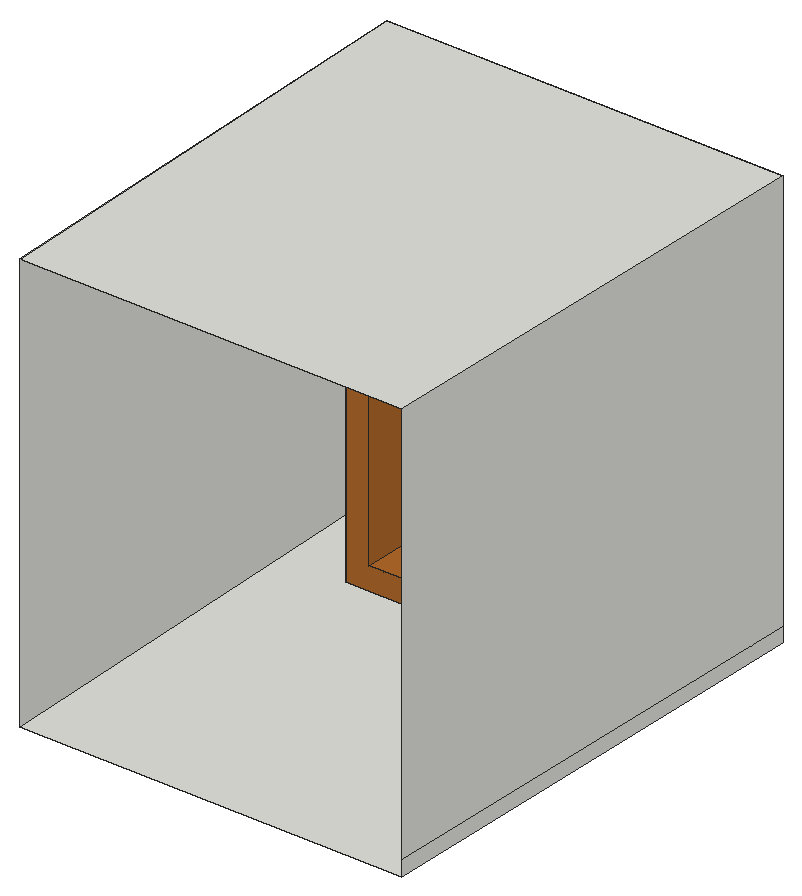
# SketchUp Ruby script. Lengths in inches.
U = 1.inch
M = Sketchup.active_model
def pt(a) = Geom::Point3d.new(a.map { |v| v * U })
def face(e, loops, mat)
  f = e.add_face(loops[0].map { |a| pt(a) })
  loops[1..].each { |l| e.add_face(l.map { |a| pt(a) }).erase! }
  f.material = f.back_material = mat if mat
  f
end
# faces: each face lists its corners as indices into pts; further lists are holes
def faces(e, pts, list, mat = nil) = list.each { |f| face(e, (f[0].is_a?(Array) ? f : [f]).map { |l| l.map { |i| pts[i] } }, mat) }
# xy, xz, yz: faces in a plane at the given z, y or x. An outline is a flat list of corners, or four numbers for a rectangle; further outlines are holes
def ring(l) = l.size == 4 ? [[l[0], l[1]], [l[2], l[1]], [l[2], l[3]], [l[0], l[3]]] : l.each_slice(2).to_a
def flat(e, list, mat, &to3) = list.each { |f| face(e, (f[0].is_a?(Array) ? f : [f]).map { |l| ring(l).map { |u, v| to3.(u, v) } }, mat) }
def xy(e, z, list, mat = nil) = flat(e, list, mat) { |x, y| [x, y, z] }
def xz(e, y, list, mat = nil) = flat(e, list, mat) { |x, z| [x, y, z] }
def yz(e, x, list, mat = nil) = flat(e, list, mat) { |y, z| [x, y, z] }
def lines(e, pts, list) = list.each { |a, b| e.add_line(pt(pts[a]), pt(pts[b])) }
# prism: a flat outline (further loops are holes) pulled along v
def prism(e, loops, v, mat = nil)
  f = face(e, loops, mat); d = Geom::Vector3d.new(v.map { |x| x * U })
  f.pushpull(f.normal.samedirection?(d) ? d.length : -d.length)
end
def box(e, o, s, mat = nil) = prism(e, [[o, [o[0] + s[0], o[1], o[2]], [o[0] + s[0], o[1] + s[1], o[2]], [o[0], o[1] + s[1], o[2]]]], [0, 0, s[2]], mat)
def at(x, y, z, deg = 0) = Geom::Transformation.translation(pt([x, y, z])) * Geom::Transformation.rotation(ORIGIN, Z_AXIS, deg.degrees)
def axes(o, x, y, z) = Geom::Transformation.new([*x, 0, *y, 0, *z, 0, *pt(o).to_a, 1])
def part(name) = M.definitions.add(name)
# library, detail: a bought-in or finely detailed component or shape, given as its bounding box
def library(name, o, s) = part(name).tap { |d| box(d.entities, o, s) }
def detail(e, o, s) = box(e.add_group.entities, o, s)
def put(e, d, t, mat = nil) = e.add_instance(d, t).tap { |i| i.material = mat if mat }
def group(e, t, mat = nil) = e.add_group.tap { |g| g.transformation = t; g.material = mat if mat }.entities
root = M.entities
M.materials.add("[Field Square Tile]").color = [217, 201, 169]
M.materials.add("[Mirror 02]").color = [229, 229, 229]
M.materials.add("[Wood Bamboo]").color = [177, 105, 43]
M.materials.add("[Wood Floor Parquet]").color = [145, 89, 39]
c1 = part("Group19\#1")
p = [[0,0,0],[0,0,-10.8125],[-3.6875,0,-10.8125],[24,-11,0],[-24,-11,0],[24,11,0],
  [24,0,0],[-24,11,0],[3.6875,0,-10.8125],[-24,0,0],[0,0,-17.5]]
lines(c1.entities,p,[[0,1],[1,2],[3,4],[5,6],[7,5],[1,8],[9,0],[0,6],[8,10],[4,9],[6,3],[2,10],
  [9,7]])
c2 = part("Rectangle Light")
put(c2.entities,c1,at(0,0,0))
c3 = part("Timber post")
box(c3.entities,[0,-2,0],[2,2,84],"[Wood Bamboo]")
c4 = part("Group\#13")
put(c4.entities,c3,at(0,0,0))
c5 = library("Group\#4",[0,0,0],[15,0.9,42])
c6 = library("Group\#5",[0,0,0],[15,0.9,60])
xy(root,-6,[[3.67,0,104.23,0,104.23,125.21,0,125.21]])
xy(root,104.23,[[3.67,0,0,125.21,104.23,125.21,104.23,0]])
xz(root,125.21,[[0,-6,104.23,104.23]])
yz(root,104.23,[[0,-6,125.21,-2.16],[0,-2.16,125.21,104.23]])
p = [[3.67,0,-6],[0,125.21,-6],[0,125.21,104.23],[3.67,0,104.23]]
faces(root,p,[[0,1,2,3]])
g1 = group(root,at(24.24,113.14,0))
box(g1,[0,2,0],[48,2,84])
xz(g1,0,[[0,0,2,84],[2,0,47.75,84],[47.75,0,48,84]])
g2 = group(g1,at(-6,0,-6),"[Wood Bamboo]")
prism(g2,[[[0,2,0],[0,2,96],[60,2,96],[60,2,0]],[[6,2,90],[6,2,6],[54,2,6],[54,2,90]]],[0,-26,0])
put(g2,c2,axes([30,-13,89.99],[1,0,0],[0,-1,0],[0,0,1]))
g3 = group(g1,at(0,0,0))
put(g3,c3,at(0,0,0))
put(g1,c4,at(3,0,0))
put(g1,c4,at(6,0,0))
put(g1,c4,at(9,0,0))
put(g1,c4,at(12,0,0))
put(g1,c4,at(15.125,0,0))
g4 = group(g1,at(18.125,0,0))
put(g4,c3,at(0,0,0))
put(g1,c4,at(24.25,0,0))
put(g1,c4,at(21.25,0,0))
put(g1,c4,at(30.375,0,0))
g5 = group(g1,at(27.375,0,0))
put(g5,c3,at(0,0,0))
put(g1,c4,at(33.5,0,0))
put(g1,c4,at(36.5,0,0))
put(g1,c4,at(42.625,0,0))
put(g1,c4,at(39.625,0,0))
put(g1,c4,at(45.75,0,0))
put(root,c5,at(57.24,110.24,42))
put(root,c6,at(24.24,110.24,0))
g6 = group(root,at(32.24,110.24,4))
box(g6,[2,-8,0],[27.71,8,8],"[Wood Floor Parquet]")
g7 = group(root,at(32.24,110.24,14))
box(g7,[0,-8,0],[31.625,8,4],"[Field Square Tile]")
g8 = group(root,at(40.39,111.14,32.41))
xy(g8,0,[[6,-0.39,9.43,0]])
xy(g8,33.19,[[6,-0.39,9.43,0]])
xz(g8,-0.39,[[6,0,9.43,0,10.21,0.05,10.98,0.2,11.72,0.46,12.43,0.8,13.08,1.24,13.67,1.76,14.1875,2.35,14.62,3,14.97,3.7,15.22,4.45,15.375,5.22,15.43,6,15.43,27.19,15.375,27.97,15.22,28.74,14.97,29.49,14.62,30.19,14.1875,30.84,13.67,31.43,13.08,31.95,12.43,32.39,11.72,32.73,10.98,32.99,10.21,33.14,9.43,33.19,6,33.19,5.22,33.14,4.45,32.99,3.7,32.73,3,32.39,2.35,31.95,1.76,31.43,1.24,30.84,0.8,30.19,0.46,29.49,0.2,28.74,0.05,27.97,0,27.19,0,6,0.05,5.22,0.2,4.45,0.46,3.7,0.8,3,1.24,2.35,1.76,1.76,2.35,1.24,3,0.8,3.7,0.46,4.45,0.2,5.22,0.05]],"[Mirror 02]")
xz(g8,0,[[6,0,5.22,0.05,4.45,0.2,3.7,0.46,3,0.8,2.35,1.24,1.76,1.76,1.24,2.35,0.8,3,0.46,3.7,0.2,4.45,0.05,5.22,0,6,0,27.19,0.05,27.97,0.2,28.74,0.46,29.49,0.8,30.19,1.24,30.84,1.76,31.43,2.35,31.95,3,32.39,3.7,32.73,4.45,32.99,5.22,33.14,6,33.19,9.43,33.19,10.21,33.14,10.98,32.99,11.72,32.73,12.43,32.39,13.08,31.95,13.67,31.43,14.1875,30.84,14.62,30.19,14.97,29.49,15.22,28.74,15.375,27.97,15.43,27.19,15.43,6,15.375,5.22,15.22,4.45,14.97,3.7,14.62,3,14.1875,2.35,13.67,1.76,13.08,1.24,12.43,0.8,11.72,0.46,10.98,0.2,10.21,0.05,9.43,0]])
yz(g8,0,[[-0.39,6,0,27.19]])
yz(g8,15.43,[[-0.39,6,0,27.19]])
p = [[6,-0.39,0],[5.22,-0.39,0.05],[5.22,0,0.05],[6,0,0],[10.21,-0.39,0.05],[9.43,-0.39,0],
  [9.43,0,0],[10.21,0,0.05],[4.45,-0.39,0.2],[4.45,0,0.2],[10.98,-0.39,0.2],[10.98,0,0.2],
  [3.7,-0.39,0.46],[3.7,0,0.46],[11.72,-0.39,0.46],[11.72,0,0.46],[3,-0.39,0.8],[3,0,0.8],
  [12.43,-0.39,0.8],[12.43,0,0.8],[2.35,-0.39,1.24],[2.35,0,1.24],[13.08,-0.39,1.24],[13.08,0,1.24],
  [1.76,-0.39,1.76],[1.76,0,1.76],[13.67,-0.39,1.76],[13.67,0,1.76],[1.24,-0.39,2.35],[1.24,0,2.35],
  [14.1875,-0.39,2.35],[14.1875,0,2.35],[0.8,-0.39,3],[0.8,0,3],[14.62,-0.39,3],[14.62,0,3],
  [0.46,-0.39,3.7],[0.46,0,3.7],[14.97,-0.39,3.7],[14.97,0,3.7],[0.2,-0.39,4.45],[0.2,0,4.45],
  [15.22,-0.39,4.45],[15.22,0,4.45],[0.05,-0.39,5.22],[0.05,0,5.22],[15.375,-0.39,5.22],[15.375,0,5.22],
  [0,-0.39,6],[0,0,6],[15.43,-0.39,6],[15.43,0,6],[0,-0.39,27.19],[0.05,-0.39,27.97],
  [0.05,0,27.97],[0,0,27.19],[15.375,-0.39,27.97],[15.43,-0.39,27.19],[15.43,0,27.19],[15.375,0,27.97],
  [0.2,-0.39,28.74],[0.2,0,28.74],[15.22,-0.39,28.74],[15.22,0,28.74],[0.46,-0.39,29.49],[0.46,0,29.49],
  [14.97,-0.39,29.49],[14.97,0,29.49],[0.8,-0.39,30.19],[0.8,0,30.19],[14.62,-0.39,30.19],[14.62,0,30.19],
  [1.24,-0.39,30.84],[1.24,0,30.84],[14.1875,-0.39,30.84],[14.1875,0,30.84],[1.76,-0.39,31.43],[1.76,0,31.43],
  [13.67,-0.39,31.43],[13.67,0,31.43],[2.35,-0.39,31.95],[2.35,0,31.95],[13.08,-0.39,31.95],[13.08,0,31.95],
  [3,-0.39,32.39],[3,0,32.39],[12.43,-0.39,32.39],[12.43,0,32.39],[3.7,-0.39,32.73],[3.7,0,32.73],
  [11.72,-0.39,32.73],[11.72,0,32.73],[4.45,-0.39,32.99],[4.45,0,32.99],[10.98,-0.39,32.99],[10.98,0,32.99],
  [5.22,-0.39,33.14],[5.22,0,33.14],[10.21,-0.39,33.14],[10.21,0,33.14],[6,-0.39,33.19],[6,0,33.19],
  [9.43,-0.39,33.19],[9.43,0,33.19]]
faces(g8,p,[[0,1,2,3],[4,5,6,7],[1,8,9,2],[10,4,7,11],[8,12,13,9],[14,10,11,15],[12,16,17,13],[18,14,15,19],
  [16,20,21,17],[22,18,19,23],[20,24,25,21],[26,22,23,27],[24,28,29,25],[30,26,27,31],[28,32,33,29],[34,30,31,35],
  [32,36,37,33],[38,34,35,39],[36,40,41,37],[42,38,39,43],[40,44,45,41],[46,42,43,47],[44,48,49,45],[50,46,47,51],
  [52,53,54,55],[56,57,58,59],[53,60,61,54],[62,56,59,63],[60,64,65,61],[66,62,63,67],[64,68,69,65],[70,66,67,71],
  [68,72,73,69],[74,70,71,75],[72,76,77,73],[78,74,75,79],[76,80,81,77],[82,78,79,83],[80,84,85,81],[86,82,83,87],
  [84,88,89,85],[90,86,87,91],[88,92,93,89],[94,90,91,95],[92,96,97,93],[98,94,95,99],[96,100,101,97],[102,98,99,103]])
